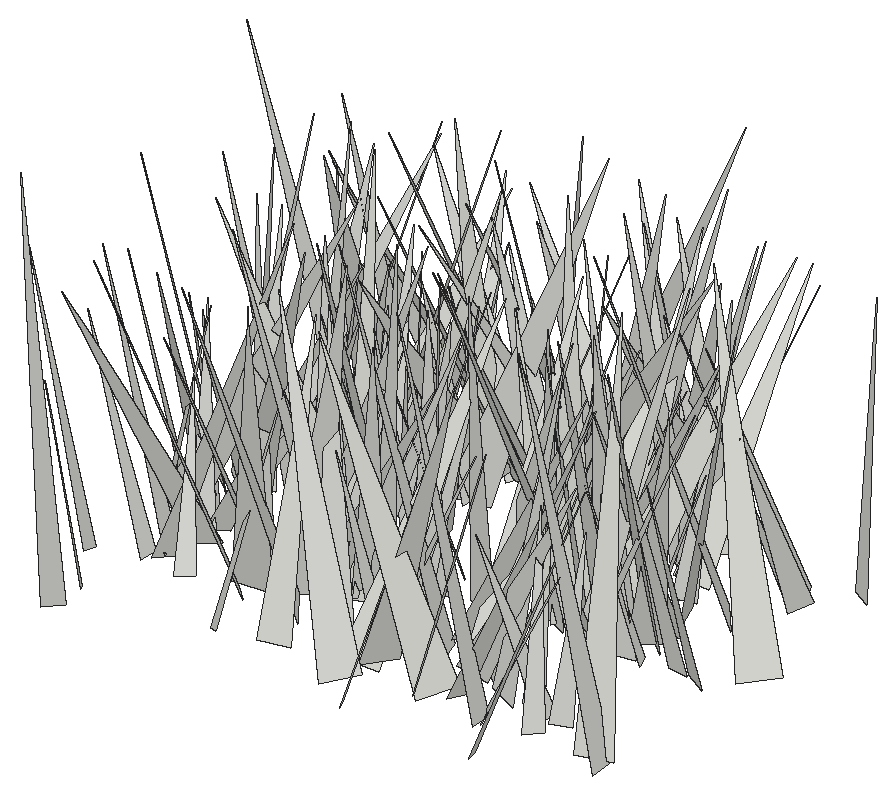
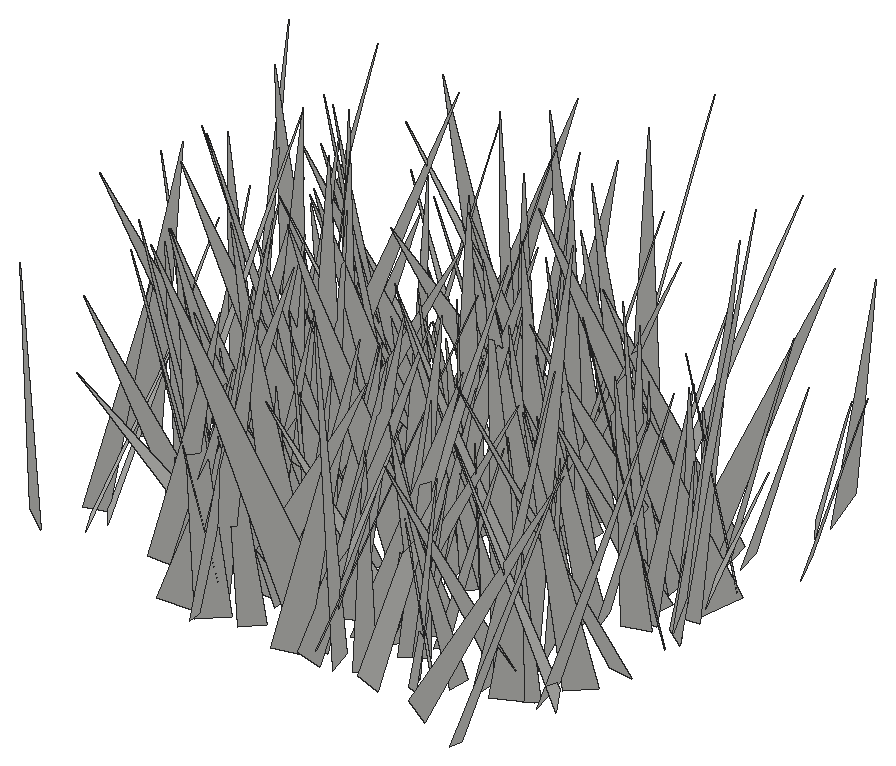
# SketchUp Ruby script. Lengths in inches.
U = 1.inch
M = Sketchup.active_model
def pt(a) = Geom::Point3d.new(a.map { |v| v * U })
def face(e, loops, mat)
  f = e.add_face(loops[0].map { |a| pt(a) })
  loops[1..].each { |l| e.add_face(l.map { |a| pt(a) }).erase! }
  f.material = f.back_material = mat if mat
  f
end
# faces: each face lists its corners as indices into pts; further lists are holes
def faces(e, pts, list, mat = nil) = list.each { |f| face(e, (f[0].is_a?(Array) ? f : [f]).map { |l| l.map { |i| pts[i] } }, mat) }
# xy, xz, yz: faces in a plane at the given z, y or x. An outline is a flat list of corners, or four numbers for a rectangle; further outlines are holes
def ring(l) = l.size == 4 ? [[l[0], l[1]], [l[2], l[1]], [l[2], l[3]], [l[0], l[3]]] : l.each_slice(2).to_a
def flat(e, list, mat, &to3) = list.each { |f| face(e, (f[0].is_a?(Array) ? f : [f]).map { |l| ring(l).map { |u, v| to3.(u, v) } }, mat) }
def xy(e, z, list, mat = nil) = flat(e, list, mat) { |x, y| [x, y, z] }
def xz(e, y, list, mat = nil) = flat(e, list, mat) { |x, z| [x, y, z] }
def yz(e, x, list, mat = nil) = flat(e, list, mat) { |y, z| [x, y, z] }
def lines(e, pts, list) = list.each { |a, b| e.add_line(pt(pts[a]), pt(pts[b])) }
# prism: a flat outline (further loops are holes) pulled along v
def prism(e, loops, v, mat = nil)
  f = face(e, loops, mat); d = Geom::Vector3d.new(v.map { |x| x * U })
  f.pushpull(f.normal.samedirection?(d) ? d.length : -d.length)
end
def box(e, o, s, mat = nil) = prism(e, [[o, [o[0] + s[0], o[1], o[2]], [o[0] + s[0], o[1] + s[1], o[2]], [o[0], o[1] + s[1], o[2]]]], [0, 0, s[2]], mat)
def at(x, y, z, deg = 0) = Geom::Transformation.translation(pt([x, y, z])) * Geom::Transformation.rotation(ORIGIN, Z_AXIS, deg.degrees)
def axes(o, x, y, z) = Geom::Transformation.new([*x, 0, *y, 0, *z, 0, *pt(o).to_a, 1])
def part(name) = M.definitions.add(name)
# library, detail: a bought-in or finely detailed component or shape, given as its bounding box
def library(name, o, s) = part(name).tap { |d| box(d.entities, o, s) }
def detail(e, o, s) = box(e.add_group.entities, o, s)
def put(e, d, t, mat = nil) = e.add_instance(d, t).tap { |i| i.material = mat if mat }
def group(e, t, mat = nil) = e.add_group.tap { |g| g.transformation = t; g.material = mat if mat }.entities
root = M.entities
c1 = part("fur_instance\#9")
p = [[0.8125,0,1.79],[0.67,-0.02,1.48],[0,-0.11,0],[0,0.11,0]]
faces(c1.entities,p,[[0,1,2,3]])
put(root,c1,axes([66.11,360.4375,-27.1],[-3.1769,-1.92196,0.83625],[-2.09296,2.82701,-1.45378],[-0.11299,1.67333,3.4166]))
put(root,c1,axes([66.16,358.79,-27.1],[-7.80069,-0.47128,0.71432],[-0.70737,7.23754,-2.94972],[0.48165,2.99651,7.23686]))
put(root,c1,axes([73.01,364.16,-27.1],[-6.10663,-5.12788,1.30944],[-4.81653,6.21333,1.86984],[2.19336,-0.63253,7.75176]))
put(root,c1,axes([80.8,362.37,-27.1],[-5.74656,4.30747,2.03787],[4.75581,5.38477,2.02895],[0.29923,-2.86007,6.88916]))
put(root,c1,axes([84.56,359.59,-27.1],[4.68389,2.5085,0.46697],[2.25732,-4.52881,1.68637],[-1.1896,1.28326,5.03861]))
put(root,c1,axes([83.1,362.13,-27.1],[3.88446,1.51086,0.00017],[1.46105,-3.75628,-1.06181],[0.38475,-0.98965,4.03042]))
put(root,c1,axes([77.45,361,-27.1],[-6.20404,3.776,0.73856],[3.82283,6.20814,0.37243],[0.43544,-0.70326,7.25325]))
put(root,c1,axes([77.75,362.82,-27.1],[6.355,-3.28716,0.66061],[-3.33311,-6.3472,0.48096],[-0.36352,0.73183,7.13864]))
put(root,c1,axes([70.61,363.84,-27.1],[-5.16383,-5.19186,0.43743],[-5.2089,5.15828,-0.26709],[0.11856,0.49863,7.31773]))
put(root,c1,axes([70.88,364.25,-27.1],[2.24537,-6.9608,0.71668],[-6.96969,-2.1575,0.8813],[0.62434,0.94895,7.26069]))
put(root,c1,axes([88.74,361.8,-27.1],[-7.60093,-1.69118,1.08047],[-1.85126,7.54274,-1.21718],[0.77483,1.43129,7.69108]))
put(root,c1,axes([85,363.36,-27.1],[0.84597,-3.78981,1.14812],[-3.67965,-1.18614,-1.20406],[-1.46323,0.79177,3.69169]))
put(root,c1,axes([79.92,362.22,-27.1],[4.69401,2.26049,0.88712],[2.32694,-4.7392,-0.23643],[-0.69438,-0.60059,5.20458]))
put(root,c1,axes([83.23,361.74,-27.1],[-7.26619,-2.16018,0.91047],[-2.32448,7.02333,-1.88745],[0.30351,2.07347,7.34176]))
put(root,c1,axes([78.58,359.6875,-27.1],[6.47169,4.71895,0.84374],[4.29058,-6.33416,2.51645],[-2.13805,1.57262,7.60387]))
put(root,c1,axes([71.67,361.01,-27.1],[2.88186,3.44939,0.31018],[3.15851,-2.7832,1.60537],[-1.42067,0.8094,4.19835]))
put(root,c1,axes([85.27,362.2,-27.1],[-3.68366,1.92684,0.76086],[1.83141,3.75443,-0.64122],[0.96827,0.22919,4.10742]))
put(root,c1,axes([74.02,361.52,-27.1],[-1.14776,6.0133,0.84328],[6.0716,1.14805,0.07727],[0.08148,-0.84289,6.12137]))
put(root,c1,axes([67.57,365.76,-27.1],[0.6668,-6.36542,0.43774],[-6.10772,-0.7641,-1.80742],[-1.84553,0.22889,6.13974]))
put(root,c1,axes([85.68,363.26,-27.1],[-1.6026,3.32948,1.45838],[3.48573,1.8596,-0.41502],[1.03054,-1.11225,3.67172]))
put(root,c1,axes([80.87,364.23,-27.1],[2.62599,-5.06265,0.78885],[-4.77605,-2.09765,2.43674],[1.85526,1.76578,5.15641]))
put(root,c1,axes([76.58,364.39,-27.1],[-3.79793,-0.43925,1.06155],[-0.29859,3.91782,0.55288],[1.10936,-0.44932,3.78306]))
put(root,c1,axes([64.625,362.81,-27.1],[-5.41168,-1.42657,0.35166],[-1.45652,5.03228,-1.99993],[-0.1932,2.0214,5.22701]))
put(root,c1,axes([66.51,363.76,-27.1],[-4.63616,-0.58897,0.33378],[-0.62989,4.59941,-0.63319],[0.24806,0.67142,4.63033]))
put(root,c1,axes([83.89,363.95,-27.1],[-2.42915,2.39744,1.43013],[2.49267,2.71628,-0.31959],[1.25681,-0.75355,3.39799]))
put(root,c1,axes([81.48,362.66,-27.1],[6.28882,0.29269,0.74734],[0.08478,-6.11246,1.68051],[-0.79813,1.65699,6.06719]))
put(root,c1,axes([72.62,365.04,-27.1],[5.72788,-5.11466,1.67521],[-5.30647,-5.77538,0.51083],[-0.89854,1.50329,7.66207]))
put(root,c1,axes([74.9375,363.86,-27.1],[1.5886,-5.12639,3.23902],[-5.9044,-2.07062,-0.3813],[-1.38174,2.95423,5.35333]))
put(root,c1,axes([68.4375,363.41,-27.1],[-2.65941,2.49787,0.36396],[2.46932,2.68404,-0.37765],[0.52369,0.0288,3.62894]))
put(root,c1,axes([82.79,363.56,-27.1],[2.70818,5.99392,1.73773],[6.22026,-2.74585,-0.22279],[-0.5051,-1.67756,6.57356]))
put(root,c1,axes([88.07,362.11,-27.1],[-0.32528,8.12923,0.88129],[8.06717,0.17507,1.36272],[-1.33486,-0.92294,8.0208]))
put(root,c1,axes([69.37,366.41,-27.1],[-3.58338,-3.97137,0.418],[-3.89573,3.60001,0.80641],[0.87736,-0.23507,5.28792]))
put(root,c1,axes([74.7,366.11,-27.1],[2.07468,-5.92746,1.15005],[-6.03286,-1.98482,0.6533],[0.24901,1.299,6.24598]))
put(root,c1,axes([76.66,364.81,-27.1],[3.8277,2.64651,0.3376],[2.6435,-3.68235,-1.10521],[0.36045,-1.09797,4.52038]))
put(root,c1,axes([66.93,364.55,-27.1],[-5.59376,-1.56322,0.76508],[-1.67452,5.53596,-0.93185],[0.47433,1.10847,5.73284]))
put(root,c1,axes([79.26,364.92,-27.1],[-7.24522,-3.15461,1.03201],[-3.28219,7.17812,-1.10079],[0.49381,1.42581,7.82516]))
put(root,c1,axes([73.9375,365.2,-27.1],[-6.93543,-2.32629,0.88421],[-2.41004,6.93097,-0.66862],[0.62063,0.91853,7.28456]))
put(root,c1,axes([75.76,365.47,-27.1],[-2.07525,-6.86081,3.30693],[-7.48887,2.46229,0.40886],[1.38687,3.02978,7.15613]))
put(root,c1,axes([72.81,365.82,-27.1],[4.53332,-3.78068,0.06575],[-3.6354,-4.32956,1.69931],[1.04008,1.34544,5.65304]))
put(root,c1,axes([65.54,368.39,-27.1],[-1.80775,-6.68688,0.47497],[-6.40102,1.86794,1.93536],[1.9917,-0.06601,6.65106]))
put(root,c1,axes([77.28,362.25,-27.1],[-4.67484,5.38464,0.57126],[4.73589,4.43174,-3.01759],[2.62527,1.59378,6.46085]))
put(root,c1,axes([65.61,365.55,-27.1],[3.51843,3.11531,1.14482],[3.25687,-3.56198,-0.31656],[-0.63919,-1.00114,4.68874]))
put(root,c1,axes([84.57,366.15,-27.1],[-3.5972,0.42819,0.55364],[0.48536,3.61469,0.35791],[0.50428,-0.42464,3.60487]))
put(root,c1,axes([67.03,364.01,-27.1],[6.5419,0.41912,1.71437],[-0.23349,-6.31856,2.43568],[-1.74935,2.41069,6.08602]))
put(root,c1,axes([72.625,366.55,-27.1],[-4.98307,4.13485,3.06586],[4.6284,5.46651,0.15019],[2.25263,-2.08511,6.47344]))
put(root,c1,axes([83.41,368.04,-27.1],[-4.28269,-7.03673,0.88853],[-7.06243,4.13524,-1.29164],[-0.65353,1.42504,8.13564]))
put(root,c1,axes([73.49,364.96,-27.1],[1.79121,4.66243,0.42191],[4.67903,-1.79759,0.00003],[-0.15134,-0.39383,4.99466]))
put(root,c1,axes([73.9375,366.41,-27.1],[3.63408,5.21962,1.38175],[5.32326,-3.18476,-1.96987],[0.90365,-2.23003,6.04736]))
put(root,c1,axes([73.88,368.55,-27.1],[-3.21608,-6.87634,1.40534],[-6.91778,3.36666,0.64196],[1.18463,0.99184,7.56406]))
put(root,c1,axes([69.6,365.53,-27.1],[-4.54245,-0.30979,1.16713],[-0.64985,4.4561,-1.34644],[1.01777,1.46262,4.34936]))
put(root,c1,axes([67.3,368.48,-27.1],[7.07591,-3.11018,0.05148],[-3.09924,-7.06002,-0.5432],[-0.26559,-0.47663,7.71016]))
put(root,c1,axes([67.09,366.15,-27.1],[-1.17354,4.22506,1.16991],[4.38332,1.15287,0.2334],[0.0799,-1.19029,4.3788]))
put(root,c1,axes([79.09,366.1,-27.1],[5.6454,-1.61471,0.55375],[-1.70236,-5.46688,1.41409],[-0.12614,1.5134,5.69896]))
put(root,c1,axes([78.53,368.125,-27.1],[5.01746,5.30698,2.27397],[5.71554,-4.13917,-2.95123],[0.81705,-3.63499,6.68051]))
put(root,c1,axes([76.23,367.54,-27.1],[4.61817,-3.87726,2.02523],[-4.05143,-4.90172,-0.14567],[-1.64942,1.18414,6.02822]))
put(root,c1,axes([84.08,370.39,-27.1],[-3.7888,-7.35051,1.42507],[-6.56657,4.02946,3.32556],[3.59735,-0.38635,7.57137]))
put(root,c1,axes([81.83,364.23,-27.1],[4.6203,4.92142,0.32663],[4.69042,-4.52255,1.79463],[-1.52544,1.00021,6.50745]))
put(root,c1,axes([83.48,367.18,-27.1],[5.31801,3.62577,0.57345],[3.65614,-5.14142,-1.39812],[0.32822,-1.47507,6.28273]))
put(root,c1,axes([65.12,369.69,-27.1],[-4.90749,-6.3294,1.61985],[-6.13533,5.16095,1.5783],[2.24565,0.26836,7.85199]))
put(root,c1,axes([87.46,368.66,-27.1],[-1.94034,-4.30134,0.80925],[-4.30819,2.03312,0.47669],[0.77193,0.53502,4.69459]))
put(root,c1,axes([71.875,366.33,-27.1],[6.69974,-1.69034,1.74311],[-2.11177,-6.58131,1.73465],[-1.19837,2.1474,6.68841]))
put(root,c1,axes([80.61,368.97,-27.1],[-1.45623,-6.82166,1.9418],[-6.84757,1.86878,1.42991],[1.84835,1.54881,6.82723]))
put(root,c1,axes([70.27,365.55,-27.1],[-6.71472,0.14595,1.05093],[-0.21339,6.41005,-2.25365],[1.03933,2.25902,6.32691]))
put(root,c1,axes([72.54,368.42,-27.1],[-7.38136,0.22251,0.33251],[0.26326,7.32737,0.9407],[0.30128,-0.95116,7.32455]))
put(root,c1,axes([66.55,369.48,-27.1],[-0.44013,-4.40012,0.04518],[-4.35564,0.44209,0.62427],[0.62566,-0.01764,4.37779]))
put(root,c1,axes([78.22,368.14,-27.1],[-1.72933,-6.01967,2.37326],[-6.41752,1.90965,0.16749],[0.82719,2.23073,6.26091]))
put(root,c1,axes([65.21,367.02,-27.1],[6.5519,-4.81181,0.9912],[-4.80718,-5.93833,2.94799],[1.01342,2.94042,7.57563]))
put(root,c1,axes([82.35,368.91,-27.1],[4.90048,2.76624,3.25214],[3.64641,-5.28694,-0.99757],[-2.22086,-2.5767,5.5382]))
put(root,c1,axes([74.45,366.11,-27.1],[-5.1152,1.11044,1.16629],[0.73583,5.06638,-1.59654],[1.43244,1.36283,4.98492]))
put(root,c1,axes([76.2,367.125,-27.1],[1.29664,4.3065,0.97913],[4.41517,-1.23995,-0.39328],[0.1042,-1.05001,4.48024]))
put(root,c1,axes([75.55,367.87,-27.1],[-4.97388,0.03891,0.99351],[0.0174,5.07103,-0.11152],[0.99411,0.10595,4.97278]))
put(root,c1,axes([75.82,369.91,-27.1],[-3.10311,-4.08719,0.56583],[-3.96021,3.14894,1.02739],[1.15846,-0.18348,5.02781]))
put(root,c1,axes([86.49,368.88,-27.1],[-1.41742,-4.71426,1.18858],[-4.85717,1.31918,-0.56008],[-0.21176,1.29675,4.89077]))
put(root,c1,axes([80.7,367.18,-27.1],[3.10796,2.24348,0.34109],[2.21254,-3.12436,0.38987],[-0.50422,0.11876,3.81322]))
put(root,c1,axes([82.67,369.61,-27.1],[-2.15861,-6.19615,1.53511],[-6.31129,2.3146,0.46773],[0.95736,1.28794,6.5447]))
put(root,c1,axes([65.81,367.1,-27.1],[-4.45593,-2.02584,0.38216],[-1.95722,3.87117,-2.29973],[-0.64758,2.23951,4.32095]))
put(root,c1,axes([71.12,371.07,-27.1],[-1.84691,-6.18778,0.26193],[-5.9057,1.84189,1.87043],[1.86547,-0.29517,6.18071]))
put(root,c1,axes([80.29,365.89,-27.1],[-2.04424,6.85145,0.72305],[6.79433,2.1298,-0.97223],[1.1412,-0.40704,7.08351]))
put(root,c1,axes([84.32,369.78,-27.1],[4.15858,-4.6502,0.45845],[-4.67236,-4.14601,0.32855],[-0.05962,0.56087,6.22978]))
put(root,c1,axes([85.04,368.67,-27.1],[-3.24657,-1.58505,0.39086],[-1.61743,3.24104,-0.29141],[0.22149,0.43432,3.60107]))
put(root,c1,axes([66.27,367.85,-27.1],[1.10778,3.32388,1.25845],[3.28018,-1.46364,0.97838],[-1.36832,-0.8177,3.36424]))
put(root,c1,axes([74.29,365.78,-27.1],[0.27633,8.1596,0.76138],[7.93766,-0.45592,2.00518],[-2.0377,-0.66947,7.91421]))
put(root,c1,axes([67.32,366.7,-27.1],[6.04009,-0.71684,0.90558],[-1.00409,-5.64184,2.23115],[-0.57074,2.3393,5.65849]))
put(root,c1,axes([75.07,368.37,-27.1],[3.97041,-1.42005,1.05601],[-1.57618,-4.01704,0.5243],[-0.80459,0.86179,4.18399]))
put(root,c1,axes([82.32,370.46,-27.1],[3.11086,-6.46121,1.0779],[-6.53922,-3.13316,0.09147],[-0.38422,1.01124,7.17051]))
put(root,c1,axes([84.72,370.84,-27.1],[-0.49515,-5.81147,0.35136],[-5.82208,0.49376,-0.03799],[-0.0081,0.35331,5.8324]))
put(root,c1,axes([84.35,368.52,-27.1],[-0.90978,-4.59674,2.27002],[-5.08569,0.51819,-0.98893],[-0.64715,2.39002,4.58036]))
put(root,c1,axes([66.72,368.43,-27.1],[3.29977,-2.51906,0.3221],[-2.3698,-2.86445,1.87534],[0.91296,1.66948,3.70368]))
put(root,c1,axes([65.06,369.66,-27.1],[-2.14945,-3.42966,1.0737],[-3.50191,2.27993,0.27214],[0.80747,0.75821,4.03839]))
put(root,c1,axes([73.53,367.73,-27.1],[-4.06355,5.05875,1.67662],[5.05755,4.32523,-0.79246],[1.68023,-0.78477,6.44014]))
put(root,c1,axes([83.28,367.45,-27.1],[2.96798,6.81466,1.03357],[6.887,-2.97737,-0.1458],[-0.27767,-1.00619,7.4315]))
put(root,c1,axes([71.31,366.93,-27.1],[2.8075,7.47142,1.47372],[7.21104,-3.11318,2.04573],[-2.44844,-0.60171,7.71486]))
put(root,c1,axes([67.65,368.25,-27.1],[-6.13991,-1.94187,2.86824],[-2.65031,6.39227,-1.34568],[2.23013,2.25037,6.2975]))
put(root,c1,axes([68.13,370.53,-27.1],[4.67852,-1.7119,0.20248],[-1.71617,-4.68064,0.08066],[-0.16239,0.14538,4.98123]))
put(root,c1,axes([80.99,370.98,-27.1],[-3.56669,-5.90918,0.59479],[-5.71236,3.22345,-2.22975],[-1.62517,1.63841,6.53207]))
put(root,c1,axes([74.39,370.1,-27.1],[4.38059,2.58911,2.20412],[2.75267,-4.81057,0.18002],[-1.99611,-0.9519,5.08534]))
put(root,c1,axes([81.25,369.4375,-27.1],[-7.16118,3.19135,1.99245],[3.1192,7.43157,-0.69239],[2.1036,-0.15533,7.80947]))
put(root,c1,axes([66.59,370.02,-27.1],[-1.35199,5.16754,1.66066],[5.39955,1.4549,-0.13134],[0.55327,-1.57128,5.33986]))
put(root,c1,axes([73.99,371.21,-27.1],[5.32416,0.8497,1.29821],[1.01973,-5.41351,-0.63884],[-1.1694,-0.85204,5.35356]))
put(root,c1,axes([70.57,372.29,-27.1],[4.90607,-3.46037,0.24315],[-3.44997,-4.91123,-0.28332],[-0.36191,-0.09172,5.99695]))
put(root,c1,axes([72.83,371.375,-27.1],[2.7967,-3.72992,1.22325],[-3.91864,-2.74089,0.60164],[-0.23004,1.34365,4.62297]))
put(root,c1,axes([85.49,373.08,-27.1],[-6.16047,-5.25921,0.96963],[-5.25018,6.22911,0.42963],[1.01736,0.29959,8.08864]))
put(root,c1,axes([67.79,370.5,-27.1],[-6.22819,-1.34042,0.61243],[-1.44458,6.07908,-1.38568],[0.29149,1.48668,6.21828]))
put(root,c1,axes([77.65,374.06,-27.1],[-1.30326,-6.4856,0.41929],[-6.05179,1.36694,2.33336],[2.36951,-0.07596,6.19006]))
put(root,c1,axes([72.81,375.53,-27.1],[6.08431,-4.17162,0.61258],[-3.3903,-5.47976,-3.64343],[-2.50671,-2.71408,6.41457]))
put(root,c1,axes([89.14,370.2,-27.1],[-5.24663,5.623,0.95369],[5.70188,5.20042,0.70642],[0.12741,-1.17997,7.65808]))
put(root,c1,axes([65.54,369.93,-27.1],[4.64173,5.41011,1.53464],[5.42173,-4.8336,0.64123],[-1.49305,-0.73288,7.09956]))
put(root,c1,axes([82.8,372.3,-27.1],[3.70621,1.73352,0.50221],[1.78343,-3.34171,-1.62653],[0.27688,-1.67963,3.75439]))
put(root,c1,axes([69.34,370.35,-27.1],[-4.14484,-0.82966,2.07391],[-1.4546,4.32013,-1.17886],[1.69516,1.67847,4.05935]))
put(root,c1,axes([84.28,372.09,-27.1],[6.26752,1.77798,1.53658],[2.00319,-6.33057,-0.84565],[-1.22862,-1.25168,6.45971]))
put(root,c1,axes([77.41,372.59,-27.1],[3.81653,-4.78014,0.36891],[-4.62204,-3.54318,1.90641],[1.2738,1.46558,5.81217]))
put(root,c1,axes([78.375,371.56,-27.1],[-1.43576,4.62376,1.24523],[4.74317,1.1948,1.0324],[-0.65727,-1.47798,4.73019]))
put(root,c1,axes([80.45,372.4,-27.1],[5.56558,-2.4926,0.3103],[-2.49513,-5.39934,1.38077],[0.28926,1.38533,5.93988]))
put(root,c1,axes([77.3,374.16,-27.1],[-3.93498,0.71077,2.15609],[1.47172,4.08376,1.33974],[1.72857,-1.85895,3.76754]))
put(root,c1,axes([76.67,373.11,-27.1],[6.17977,-5.38552,0.13557],[-5.06059,-5.73249,2.95646],[1.84733,2.31224,7.64543]))
put(root,c1,axes([71.3,372.13,-27.1],[2.20928,6.37096,1.50715],[6.50914,-1.9672,-1.22586],[0.70121,-1.81177,6.63078]))
put(root,c1,axes([78.35,374.06,-27.1],[0.55845,-3.67703,0.59896],[-3.72525,-0.55803,0.04757],[-0.0423,0.59936,3.71889]))
put(root,c1,axes([83.42,373.0625,-27.1],[-1.45732,3.49071,1.72371],[3.67662,1.83923,-0.61623],[1.28012,-1.30851,3.73217]))
put(root,c1,axes([82.125,371.22,-27.1],[-6.70082,0.16595,0.10129],[0.12128,6.29761,-2.29436],[0.15195,2.29157,6.29797]))
put(root,c1,axes([66.8125,376.81,-27.1],[7.11754,-4.23376,0.53848],[-3.90576,-6.88369,-2.49681],[-1.7204,-1.88792,7.89621]))
put(root,c1,axes([81.8,371.26,-27.1],[-0.75445,7.6495,1.46212],[7.18414,1.25072,-2.83648],[3.00677,-1.06897,7.14412]))
put(root,c1,axes([73.04,374.14,-27.1],[-4.43499,0.78648,1.49873],[1.10021,4.53377,0.87655],[1.28619,-1.16631,4.41807]))
put(root,c1,axes([80.39,372.14,-27.1],[-1.23415,4.06964,0.18802],[4.01431,1.18128,0.78126],[-0.69473,-0.40381,4.18028]))
put(root,c1,axes([87,375.23,-27.1],[3.36953,-3.09183,0.80409],[-2.80421,-3.42236,-1.4084],[-1.53048,-0.53643,4.35081]))
put(root,c1,axes([70.37,371.53,-27.1],[6.70956,3.50603,1.11128],[3.28027,-6.75003,1.49074],[-1.66343,0.8308,7.42214]))
put(root,c1,axes([86.29,375.44,-27.1],[-4.87517,-3.87645,0.62854],[-3.83008,4.91477,0.6039],[0.86741,-0.08574,6.19915]))
put(root,c1,axes([68.71,374.99,-27.1],[3.22144,-2.0672,0.86258],[-1.86043,-3.31076,-0.98626],[-1.24746,-0.40075,3.69841]))
put(root,c1,axes([80.44,372.9375,-27.1],[3.75823,0.40452,0.85087],[0.18545,-3.74836,0.96295],[-0.9237,0.89332,3.65522]))
put(root,c1,axes([80.23,373.12,-27.1],[-3.57041,1.71359,0.7726],[1.61509,3.64514,-0.62093],[0.96166,0.24019,3.91135]))
put(root,c1,axes([71.13,375.46,-27.1],[-3.68775,-0.43694,1.2324],[0.03671,3.65173,1.40455],[1.30705,-1.33536,3.43768]))
put(root,c1,axes([78.8125,374.01,-27.1],[3.29309,2.39527,0.08068],[2.3726,-3.23886,-0.68467],[0.3385,-0.60058,4.0141]))
put(root,c1,axes([67.92,373.24,-27.1],[-5.24858,-0.93793,1.2858],[-1.33069,5.01688,-1.77222],[0.87308,2.00792,5.02857]))
put(root,c1,axes([72.91,373.89,-27.1],[5.54256,-5.39998,2.31392],[-5.86744,-4.92827,2.55329],[0.29519,3.43313,7.30483]))
put(root,c1,axes([76.33,374.78,-27.1],[-4.97411,1.9133,1.24146],[2.05101,5.05519,0.42681],[0.99764,-0.85328,5.31228]))
put(root,c1,axes([74.58,378.14,-27.1],[-5.86145,-3.99032,0.23805],[-3.68658,5.55942,2.41617],[1.54546,-1.87245,6.66644]))
put(root,c1,axes([75.2,375.94,-27.1],[3.86572,-4.28586,2.24353],[-4.19582,-4.39988,-1.17556],[-2.40771,0.7863,5.6507]))
put(root,c1,axes([81.4,375.62,-27.1],[-6.84332,-0.22544,2.15666],[-0.013,7.14388,0.70553],[2.16837,-0.66867,6.81058]))
put(root,c1,axes([65.02,372.86,-27.1],[2.4491,6.4359,0.09226],[6.32974,-2.3903,-1.28384],[1.16776,-0.54137,6.7654]))
put(root,c1,axes([78.89,372.78,-27.1],[-1.68385,4.77561,0.18208],[4.53538,1.65768,-1.53538],[1.50664,0.34725,4.82539]))
put(root,c1,axes([69.54,375.1,-27.1],[3.09242,2.58599,1.68004],[2.84079,-3.31463,-0.12697],[-1.19992,-1.18273,4.02918]))
put(root,c1,axes([66.19,376.47,-27.1],[-0.42992,-4.68733,0.89248],[-4.33891,0.75688,1.88505],[1.98531,0.63912,4.31306]))
put(root,c1,axes([82.04,375.66,-27.1],[4.94298,-3.20176,1.42299],[-3.34359,-5.04595,0.26096],[-1.0472,0.99819,5.88356]))
put(root,c1,axes([73.31,376.11,-27.1],[-3.41079,-4.86692,0.40111],[-4.72199,3.16213,-1.78467],[-1.24525,1.33989,5.66881]))
put(root,c1,axes([81.04,372.49,-27.1],[-5.5806,3.5391,0.90465],[3.04631,5.42049,-2.4135],[2.01583,1.60617,6.15169]))
put(root,c1,axes([65.36,374.72,-27.1],[2.82826,-4.43632,2.67471],[-5.15951,-2.68482,1.00262],[-0.46309,2.81866,5.16476]))
put(root,c1,axes([86.58,376.2,-27.1],[-4.47388,-2.50611,0.21033],[-2.51468,4.46372,-0.30343],[0.03476,0.36756,5.119]))
put(root,c1,axes([76.38,376.02,-27.1],[-4.16703,-2.76107,2.92288],[-2.78486,5.0182,0.77013],[2.90022,0.85149,4.93909]))
put(root,c1,axes([80.46,378.86,-27.1],[3.62515,-5.36286,0.15908],[-5.03579,-3.46731,-2.13211],[-1.85105,-1.06996,6.11196]))
put(root,c1,axes([77.58,375.77,-27.1],[6.54433,-2.87567,1.841],[-3.10892,-6.66403,0.64215],[-1.41189,1.3447,7.11937]))
put(root,c1,axes([81.07,375.33,-27.1],[3.79421,5.57197,1.64798],[5.81056,-3.63804,-1.07735],[0.00109,-1.96889,6.65448]))
put(root,c1,axes([71.54,379.08,-27.1],[-3.81436,-7.20009,0.2192],[-7.12697,3.80817,1.069],[1.0467,-0.30859,8.07762]))
put(root,c1,axes([72.45,375.97,-27.1],[-6.37075,2.32719,2.17346],[2.54476,6.64308,0.34616],[1.91413,-1.08621,6.77365]))
put(root,c1,axes([79.44,374.64,-27.1],[7.05742,-1.09775,2.22467],[-1.64487,-7.09246,1.71837],[-1.85705,2.1103,6.93249]))
put(root,c1,axes([75.16,373.73,-27.1],[4.59925,2.87418,0.36346],[2.61006,-4.40682,1.82035],[-1.25721,1.36572,5.10885]))
put(root,c1,axes([68.05,376.98,-27.1],[-6.59248,-1.12335,1.64682],[-1.04061,6.79216,0.46743],[1.70031,-0.1986,6.67115]))
put(root,c1,axes([66,375.75,-27.1],[-7.51977,-1.08655,0.44758],[-1.14316,7.43533,-1.15625],[0.27218,1.20961,7.50937]))
put(root,c1,axes([73.45,376.54,-27.1],[-4.72001,4.32069,1.36462],[4.52973,4.45158,1.57294],[-0.11027,-2.07946,6.20264]))
put(root,c1,axes([71.45,376.57,-27.1],[2.88206,-3.90926,2.29022],[-4.22914,-3.29495,-0.30223],[-1.62535,1.64154,4.8474]))
put(root,c1,axes([74.39,379,-27.1],[-1.51656,-6.50321,0.08888],[-6.50028,1.51258,-0.24097],[-0.21452,0.14123,6.67335]))
put(root,c1,axes([77.62,376.41,-27.1],[3.69637,0.13401,0.11411],[0.12786,-3.69317,0.19555],[-0.12096,0.19138,3.69362]))
put(root,c1,axes([82.78,374.28,-27.1],[-1.93845,6.02083,0.54238],[5.77969,2.01278,-1.68701],[1.77192,0.02133,6.09606]))
put(root,c1,axes([80.57,376.15,-27.1],[4.17066,5.06918,1.33611],[5.23853,-4.09478,-0.81653],[-0.19883,-1.55319,6.51339]))
put(root,c1,axes([71.9375,374.96,-27.1],[-3.2921,4.67046,0.35788],[4.62081,3.30978,-0.68745],[0.76768,0.10645,5.67261]))
put(root,c1,axes([78.93,376.3,-27.1],[-3.29072,5.65648,0.59206],[5.32719,2.82602,2.60955],[-1.99181,-1.7869,6.00123]))
put(root,c1,axes([78.8125,378.79,-27.1],[1.7793,-6.50243,0.4842],[-6.28195,-1.575,1.93351],[1.74732,0.95904,6.45825]))
put(root,c1,axes([70.05,378.44,-27.1],[-2.01295,-3.23513,0.63988],[-3.06607,2.112,1.03257],[1.21439,-0.03018,3.66768]))
put(root,c1,axes([77.38,378.36,-27.1],[2.01974,-4.62687,0.27657],[-4.52399,-1.90214,1.21619],[1.00891,0.73329,4.89981]))
put(root,c1,axes([69.64,377.73,-27.1],[4.05743,2.55482,1.17911],[2.80714,-3.81746,-1.3882],[-0.19333,-1.81108,4.58942]))
put(root,c1,axes([81.21,377.97,-27.1],[3.41803,-2.18502,2.15563],[-1.95303,-4.03718,-0.99543],[-2.36786,0.1758,3.93273]))
put(root,c1,axes([72.18,378.47,-27.1],[1.68223,-3.64936,0.16027],[-3.63941,-1.65928,0.41825],[0.31341,0.31999,3.9966]))
put(root,c1,axes([75.18,379.04,-27.1],[2.93992,-5.13493,1.13143],[-5.01799,-3.12719,-1.15379],[-1.5708,0.37938,5.8034]))
put(root,c1,axes([82.6,376.73,-27.1],[-2.33709,5.71521,1.48586],[5.84354,2.00796,1.46781],[-0.85111,-1.90732,5.99759]))
put(root,c1,axes([68.98,377.125,-27.1],[3.85375,-0.57416,0.66525],[-0.65849,-3.86826,0.47595],[-0.58191,0.57487,3.8671]))
put(root,c1,axes([74.52,378.27,-27.1],[0.87067,-3.63818,0.96208],[-3.64876,-1.05785,-0.69825],[-0.92116,0.75142,3.67517]))
put(root,c1,axes([65.48,375.875,-27.1],[5.06961,3.19969,0.78256],[3.08145,-5.11429,0.94868],[-1.16407,0.39664,5.91937]))
put(root,c1,axes([78.72,378.27,-27.1],[3.57739,2.98141,0.96801],[3.07785,-3.06266,-1.94177],[0.59384,-2.08684,4.23274]))
put(root,c1,axes([79.36,378.99,-27.1],[-5.69321,-2.11736,2.09192],[-1.78965,6.04293,1.24584],[2.37833,-0.52131,5.94506]))
put(root,c1,axes([82.03,374.43,-27.1],[4.84887,3.21318,0.05137],[2.84684,-4.33809,2.62966],[-1.49084,2.16682,5.18854]))
put(root,c1,axes([67.26,376.13,-27.1],[0.04423,5.29855,0.55334],[5.02486,0.14232,-1.76445],[1.76963,-0.53655,4.99632]))
put(root,c1,axes([75.43,377.06,-27.1],[-5.24793,-3.08562,0.82091],[-3.15493,4.76816,-2.24651],[-0.49124,2.34081,5.65818]))
put(root,c1,axes([88.2,377.15,-27.1],[2.88835,4.68484,1.93004],[4.79823,-3.24275,0.69058],[-1.62782,-1.24585,5.46016]))
put(root,c1,axes([80.03,377.5,-27.1],[-2.9661,5.6248,1.68099],[5.86235,2.73802,1.18234],[-0.31135,-2.03143,6.24805]))
put(root,c1,axes([68.92,379.58,-27.1],[-2.19806,-5.17129,0.07017],[-4.98418,2.09779,-1.52836],[-1.38027,0.66005,5.4072]))
put(root,c1,axes([70.94,377.11,-27.1],[2.36274,4.29484,1.97791],[3.91667,-3.01643,1.87116],[-2.64906,-0.62918,4.53067]))
put(root,c1,axes([73.29,378.49,-27.1],[6.28919,2.00514,2.27548],[2.25266,-6.59596,-0.4138],[-2.03074,-1.10685,6.58812]))
put(root,c1,axes([66.37,380.55,-27.1],[-5.34659,-1.99732,0.9572],[-1.60106,5.21354,1.93576],[1.5304,-1.52357,5.36919]))
put(root,c1,axes([75.82,376.85,-27.1],[7.81962,-2.04899,1.63917],[-2.46618,-7.49875,2.3913],[-0.8962,2.75717,7.72182]))
